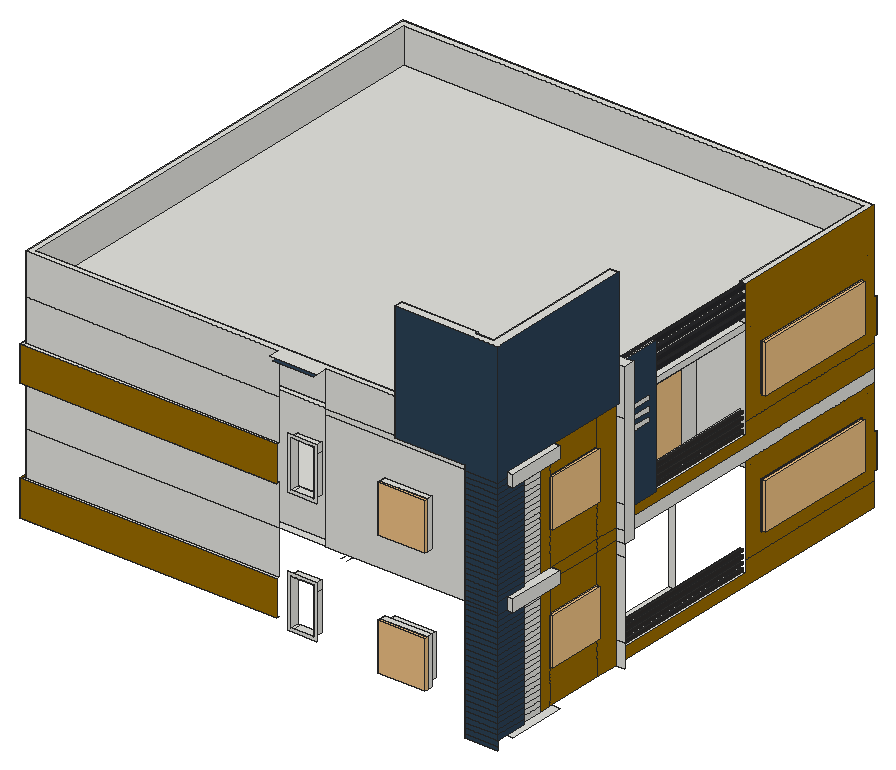
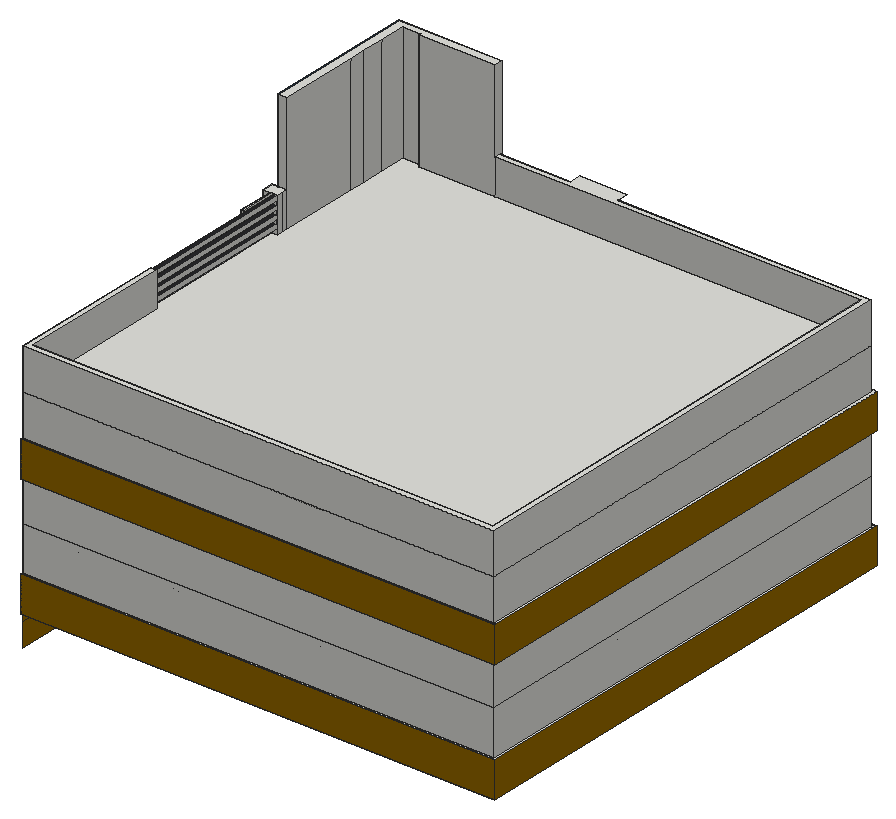
# SketchUp Ruby script. Lengths in inches.
U = 1.inch
M = Sketchup.active_model
def pt(a) = Geom::Point3d.new(a.map { |v| v * U })
def face(e, loops, mat)
  f = e.add_face(loops[0].map { |a| pt(a) })
  loops[1..].each { |l| e.add_face(l.map { |a| pt(a) }).erase! }
  f.material = f.back_material = mat if mat
  f
end
# faces: each face lists its corners as indices into pts; further lists are holes
def faces(e, pts, list, mat = nil) = list.each { |f| face(e, (f[0].is_a?(Array) ? f : [f]).map { |l| l.map { |i| pts[i] } }, mat) }
# xy, xz, yz: faces in a plane at the given z, y or x. An outline is a flat list of corners, or four numbers for a rectangle; further outlines are holes
def ring(l) = l.size == 4 ? [[l[0], l[1]], [l[2], l[1]], [l[2], l[3]], [l[0], l[3]]] : l.each_slice(2).to_a
def flat(e, list, mat, &to3) = list.each { |f| face(e, (f[0].is_a?(Array) ? f : [f]).map { |l| ring(l).map { |u, v| to3.(u, v) } }, mat) }
def xy(e, z, list, mat = nil) = flat(e, list, mat) { |x, y| [x, y, z] }
def xz(e, y, list, mat = nil) = flat(e, list, mat) { |x, z| [x, y, z] }
def yz(e, x, list, mat = nil) = flat(e, list, mat) { |y, z| [x, y, z] }
def lines(e, pts, list) = list.each { |a, b| e.add_line(pt(pts[a]), pt(pts[b])) }
# prism: a flat outline (further loops are holes) pulled along v
def prism(e, loops, v, mat = nil)
  f = face(e, loops, mat); d = Geom::Vector3d.new(v.map { |x| x * U })
  f.pushpull(f.normal.samedirection?(d) ? d.length : -d.length)
end
def box(e, o, s, mat = nil) = prism(e, [[o, [o[0] + s[0], o[1], o[2]], [o[0] + s[0], o[1] + s[1], o[2]], [o[0], o[1] + s[1], o[2]]]], [0, 0, s[2]], mat)
def at(x, y, z, deg = 0) = Geom::Transformation.translation(pt([x, y, z])) * Geom::Transformation.rotation(ORIGIN, Z_AXIS, deg.degrees)
def axes(o, x, y, z) = Geom::Transformation.new([*x, 0, *y, 0, *z, 0, *pt(o).to_a, 1])
def part(name) = M.definitions.add(name)
# library, detail: a bought-in or finely detailed component or shape, given as its bounding box
def library(name, o, s) = part(name).tap { |d| box(d.entities, o, s) }
def detail(e, o, s) = box(e.add_group.entities, o, s)
def put(e, d, t, mat = nil) = e.add_instance(d, t).tap { |i| i.material = mat if mat }
def group(e, t, mat = nil) = e.add_group.tap { |g| g.transformation = t; g.material = mat if mat }.entities
root = M.entities
M.materials.add("Carpet_04_1K").color = [43, 65, 85]
M.materials.add("D07_Ochre_Flame").color = [153, 107, 0]
M.materials.add("ThomThom - Buttons2").color = [40, 40, 43]
M.materials.add("ThomThom - Hat1").color = [48, 46, 44]
c1 = library("mesh-163",[-551.08,-704.17,-20.03],[1929.24,1401.85,86.96])
c2 = part("Group11")
put(c2.entities,c1,at(0,0,0))
xy(root,387,[[426,202,432,302]])
xy(root,396,[[486,21.29,492,21.29,492,81.29,483,81.29,483,42,486,42]])
xy(root,408,[[474,175,477,329],[480,175,483,329]])
xy(root,411,[[477,175,480,329]],"ThomThom - Hat1")
xy(root,414,[[477,175,480,329]])
xy(root,417,[[477,175,480,329]],"ThomThom - Hat1")
xy(root,420,[[369,6,417,12],[477,175,480,329]])
xy(root,423,[[372,6,414,21],[273,12,276,21],[276,12,297,21]])
xy(root,423,[[477,175,480,329]],"ThomThom - Hat1")
xy(root,426,[[477,175,480,329]])
xy(root,429,[[0,9,261,12],[0,12,3,495],[3,492,483,495]])
xy(root,429,[[477,175,480,329]],"ThomThom - Hat1")
xy(root,435,[[474,82,483,136]])
xy(root,438,[[483,347,485,474]])
xy(root,441,[[474,350,485,471]])
xy(root,465,[[372,6,414,21],[0,9,261,12],[0,12,3,495],[3,492,483,495]])
xy(root,468,[[369,6,417,12]])
xy(root,471,[[273,12,297,21]])
xy(root,477,[[474,82,483,136],[426,202,432,302]])
xy(root,483,[[474,350,485,471]])
xy(root,486,[[483,347,485,474]])
xy(root,504,[[12,21,171,169],[180,21,324,169],[330,21,474,169],[171,169,180,175],[180,169,324,175],
  [324,169,330,175],[12,175,171,329],[171,175,180,329],[180,175,324,329],[324,175,330,329],
  [330,175,426,329],[171,329,180,335],[180,329,324,335],[324,329,330,335],[330,329,426,335],
  [12,335,171,483],[171,335,180,483],[180,335,324,483],[324,335,330,483],[330,335,426,483],
  [426,335,474,483]])
xy(root,510,[[180,21,324,169],[330,21,474,169],[486,21.29,486,42,483,42,483,81.29,492,81.29,492,21.29],[12,175,426,329],[432,175,474,329],
  [12,335,474,483]])
xy(root,510,[[12,21,171,169]],"D07_Ochre_Flame")
xy(root,513,[[426,202,432,302]])
xy(root,522,[[486,21.29,492,21.29,492,81.29,483,81.29,483,42,486,42]])
xy(root,534,[[474,175,477,329],[480,175,483,329],[483,175,485.29,211]])
xy(root,537,[[477,175,480,329]],"ThomThom - Hat1")
xy(root,540,[[477,175,480,329]])
xy(root,543,[[477,175,480,329]],"ThomThom - Hat1")
xy(root,546,[[369,6,417,12],[477,175,480,329]])
xy(root,549,[[372,6,414,21],[273,12,276,21],[276,12,297,21]])
xy(root,549,[[477,175,480,329]],"ThomThom - Hat1")
xy(root,552,[[0,9,3,492],[3,9,261,12],[477,175,480,329],[0,492,483,495]])
xy(root,555,[[477,175,480,329]],"ThomThom - Hat1")
xy(root,561,[[474,82,483,136]])
xy(root,564,[[483,347,485,474]])
xy(root,567,[[474,350,485,471]])
xy(root,588,[[0,9,3,492],[3,9,261,12],[0,492,483,495]])
xy(root,591,[[372,6,414,21]])
xy(root,594,[[369,6,417,12]])
xy(root,597,[[273,12,297,21]])
xy(root,603,[[474,82,483,136],[426,202,432,302]])
xy(root,609,[[474,350,485,471]])
xy(root,612,[[483,347,485,474]])
xy(root,624,[[486,21.29,486,42,483,42,483,81.29,492,81.29,492,21.29]])
xy(root,624,[[483,21.29,486,42]],"Carpet_04_1K")
xy(root,630,[[12,21,171,169],[180,21,324,169],[330,21,474,169],[171,169,180,175],[180,169,324,175],
  [324,169,330,175],[12,175,171,329],[171,175,180,329],[180,175,324,329],[324,175,330,329],
  [330,175,426,329],[432,175,483,329],[171,329,180,335],[180,329,324,335],[324,329,330,335],
  [330,329,426,335],[12,335,171,483],[171,335,180,483],[180,335,324,483],[324,335,330,483],
  [330,335,426,483],[426,335,474,483],[171,483,180,492],[180,483,324,492],[324,483,330,492],
  [330,483,426,492]])
xy(root,636,[[459,15,477,15,477,175,483,175,483,329,477,329,477,486,9,486,9,18,459,18],[486,21.29,492,81.29]])
xy(root,636,[[381,9,453,12]],"Carpet_04_1K")
xy(root,636,[[483,21.29,486,81.29],[483,81.29,486,163]],"D07_Ochre_Flame")
xy(root,641.25,[[478,175,482,329]])
xy(root,645.5,[[478,175,482,329]],"ThomThom - Buttons2")
xy(root,649.75,[[478,175,482,329]])
xy(root,654,[[478,175,482,329]],"ThomThom - Buttons2")
xy(root,658.25,[[478,175,482,329]])
xy(root,662.5,[[478,175,482,329]],"ThomThom - Buttons2")
xy(root,666.75,[[478,175,482,329]])
xy(root,669,[[264,0,306,12]],"Carpet_04_1K")
xy(root,671,[[478,175,482,329]],"ThomThom - Buttons2")
xy(root,672,[[261,0,309,0,309,12,381,12,381,18,9,18,9,486,477,486,477,329,483,329,483,492,3,492,3,12,261,12],[477,163,492,163,492,175,485.29,175,485.29,211,483,211,483,175,477,175]])
xy(root,756,[[381,9,486,9,486,163,477,163,477,15,459,15,459,18,381,18]])
xz(root,6,[[[369,420,417,468],[372,423,414,465]],[[369,546,417,594],[372,549,414,591]]])
xz(root,9,[[453,387.3125,486,390.625],[453,390.625,486,396],[453,396,486,401.18],[453,401.18,486,406.36],[453,406.36,486,411.55],
  [453,411.55,486,416.73],[453,416.73,486,421.91],[453,421.91,486,427.09],[453,427.09,486,432.27],[453,432.27,486,437.45],
  [453,437.45,486,442.64],[453,442.64,486,447.82],[453,447.82,486,453],[453,453,486,458.18],[453,458.18,486,463.36],
  [453,463.36,486,468.55],[453,468.55,486,473.73],[453,473.73,486,478.91],[453,478.91,486,484.09],[453,484.09,486,489.27],
  [453,489.27,486,494.45],[453,494.45,486,499.64],[453,499.64,486,504.82],[453,504.82,486,510],[453,510,486,513.3125],
  [453,513.3125,486,516.625],[453,516.625,486,522],[453,522,486,527.18],[453,527.18,486,532.36],[453,532.36,486,537.55],
  [453,537.55,486,542.73],[453,542.73,486,547.91],[453,547.91,486,553.09],[453,553.09,486,558.27],[453,558.27,486,563.45],
  [453,563.45,486,568.64],[453,568.64,486,573.82],[453,573.82,486,579],[453,579,486,584.18],[453,584.18,486,589.36],
  [453,589.36,486,594.55],[453,594.55,486,599.73],[453,599.73,486,604.91],[453,604.91,486,610.09],[453,610.09,486,615.27],
  [453,615.27,486,620.45],[453,620.45,486,625.64],[453,625.64,486,630.82],[453,630.82,486,630.82,486,756,381,756,381,636,453,636]],"Carpet_04_1K")
xz(root,9,[[0,429,261,465],[0,552,261,588]],"D07_Ochre_Flame")
xz(root,12,[[[270,420,300,474],[273,423,297,471]],[3,465,261,510],[3,510,261,552],[[309,510,453,630],[369,546,417,594]],[[270,546,300,600],[273,549,297,597]],
  [3,588,261,630],[3,630,261,672],[309,630,453,636],[309,636,381,672]])
xz(root,15,[[459,636,477,756]])
xz(root,18,[[9,636,381,672],[381,636,459,756]])
xz(root,21,[[12,510,171,630],[[180,510,324,630],[273,549,297,597]],[[330,510,474,630],[372,549,414,591]]])
xz(root,21.29,[[486,510,492,522],[486,624,492,636]])
xz(root,21.29,[[483,624,486,625.64],[483,625.64,486,630.82],[483,630.82,486,636]],"Carpet_04_1K")
xz(root,42,[[483,396,486,401.18],[483,401.18,486,406.36],[483,406.36,486,411.55],[483,411.55,486,416.73],[483,416.73,486,421.91],
  [483,421.91,486,427.09],[483,427.09,486,432.27],[483,432.27,486,437.45],[483,437.45,486,442.64],[483,442.64,486,447.82],
  [483,447.82,486,453],[483,453,486,458.18],[483,458.18,486,463.36],[483,463.36,486,468.55],[483,468.55,486,473.73],
  [483,473.73,486,478.91],[483,478.91,486,484.09],[483,484.09,486,489.27],[483,489.27,486,494.45],[483,494.45,486,498],
  [483,522,486,527.18],[483,527.18,486,532.36],[483,532.36,486,537.55],[483,537.55,486,542.73],[483,542.73,486,547.91],
  [483,547.91,486,553.09],[483,553.09,486,558.27],[483,558.27,486,563.45],[483,563.45,486,568.64],[483,568.64,486,573.82],
  [483,573.82,486,579],[483,579,486,584.18],[483,584.18,486,589.36],[483,589.36,486,594.55],[483,594.55,486,599.73],
  [483,599.73,486,604.91],[483,604.91,486,610.09],[483,610.09,486,615.27],[483,615.27,486,620.45],[483,620.45,486,624]])
xz(root,42,[[483,498,486,499.64],[483,499.64,486,504.82],[483,504.82,486,510]],"Carpet_04_1K")
xz(root,81.29,[[483,510,492,522],[483,624,492,636]])
xz(root,82,[[474,435,483,477],[474,561,483,603]])
xz(root,136,[[474,435,483,477],[474,561,483,603]])
xz(root,163,[[483,396,492,420],[483,420,492,498],[483,498,492,510],[483,510,492,522],[483,522,492,546],
  [483,546,492,624],[483,624,492,624,492,672,486,672,486,636,483,636],[483,636,486,672],[477,672,486,756]])
xz(root,169,[[12,510,171,630],[171,510,180,630],[180,510,324,630],[324,510,330,630],[330,510,474,630]])
xz(root,175,[[12,510,426,630],[[432,510,432,630,483,630,483,534,480,534,480,537,477,537,477,534,474,534,474,510],[477,552,480,555],[477,540,480,543],[477,546,480,549]],[483,510,492,522],[483,522,492,534],[485.29,534,492,672],
  [[477,636,483,672],[478,666.75,482,671],[478,658.25,482,662.5],[478,649.75,482,654],[478,641.25,482,645.5]]])
xz(root,202,[[426,387,432,477],[426,513,432,603]])
xz(root,211,[[483,534,485.29,672]])
xz(root,302,[[426,387,432,477],[426,513,432,603]])
xz(root,329,[[432,504,483,510],[12,510,426,630],[[432,510,474,510,474,534,477,534,477,537,480,537,480,534,483,534,483,630,432,630],[477,540,480,543],[477,546,480,549],[477,552,480,555]],[[477,636,483,672],[478,666.75,482,671],[478,641.25,482,645.5],[478,658.25,482,662.5],[478,649.75,482,654]]])
xz(root,335,[[12,510,474,630]])
xz(root,347,[[483,438,485,486],[483,564,485,612]])
xz(root,350,[[474,441,485,483],[474,567,485,609]])
xz(root,471,[[474,441,485,483],[474,567,485,609]])
xz(root,474,[[483,438,485,486],[483,564,485,612]])
xz(root,483,[[12,510,474,630]])
xz(root,486,[[9,636,477,672]])
xz(root,492,[[3,465,483,510],[3,510,483,552],[3,588,483,630],[3,630,483,672]])
xz(root,495,[[0,429,483,465],[0,552,483,588]],"D07_Ochre_Flame")
yz(root,0,[[9,429,495,465],[9,552,495,588]],"D07_Ochre_Flame")
yz(root,3,[[12,465,492,510],[12,510,492,552],[12,588,492,630],[12,630,492,672]])
yz(root,9,[[18,636,486,672]])
yz(root,12,[[21,510,169,630],[175,510,329,630],[335,510,483,630]])
yz(root,171,[[21,510,169,630]])
yz(root,180,[[21,510,169,630]])
yz(root,273,[[12,423,21,471],[12,549,21,597]])
yz(root,297,[[12,423,21,462],[12,462,21,471],[12,549,21,588],[12,588,21,597]])
yz(root,324,[[21,510,169,630]])
yz(root,330,[[21,510,169,630]])
yz(root,369,[[6,420,12,468],[6,546,12,594]])
yz(root,372,[[6,423,21,465],[6,549,21,591]])
yz(root,381,[[9,672,18,756]])
yz(root,381,[[9,636,12,672]],"Carpet_04_1K")
yz(root,414,[[6,423,21,465],[6,549,21,591]])
yz(root,417,[[6,420,12,468],[6,546,12,594]])
yz(root,426,[[[175,510,329,630],[202,513,302,603]]])
yz(root,432,[[175,504,329,510],[175,510,199,510,199,606,305,606,305,510,329,510,329,630,175,630],[[199,510,305,606],[202,513,302,603]]])
yz(root,453,[[9,387.3125,12,390.625],[9,390.625,12,396],[9,396,12,401.18],[9,401.18,12,406.36],[9,406.36,12,411.55],
  [9,411.55,12,416.73],[9,416.73,12,421.91],[9,421.91,12,427.09],[9,427.09,12,432.27],[9,432.27,12,437.45],
  [9,437.45,12,442.64],[9,442.64,12,447.82],[9,447.82,12,453],[9,453,12,458.18],[9,458.18,12,463.36],
  [9,463.36,12,468.55],[9,468.55,12,473.73],[9,473.73,12,478.91],[9,478.91,12,484.09],[9,484.09,12,489.27],
  [9,489.27,12,494.45],[9,494.45,12,499.64],[9,499.64,12,504.82],[9,504.82,12,510],[9,510,12,513.3125],
  [9,513.3125,12,516.625],[9,516.625,12,522],[9,522,12,527.18],[9,527.18,12,532.36],[9,532.36,12,537.55],
  [9,537.55,12,542.73],[9,542.73,12,547.91],[9,547.91,12,553.09],[9,553.09,12,558.27],[9,558.27,12,563.45],
  [9,563.45,12,568.64],[9,568.64,12,573.82],[9,573.82,12,579],[9,579,12,584.18],[9,584.18,12,589.36],
  [9,589.36,12,594.55],[9,594.55,12,599.73],[9,599.73,12,604.91],[9,604.91,12,610.09],[9,610.09,12,615.27],
  [9,615.27,12,620.45],[9,620.45,12,625.64],[9,625.64,12,630.82],[9,630.82,12,636]])
yz(root,459,[[15,636,18,756]])
yz(root,474,[[[21,510,169,630],[82,561,136,603]],[175,510,329,534],[[335,510,483,630],[350,567,471,609]]])
yz(root,477,[[175,408,329,411],[175,414,329,417],[175,420,329,423],[175,426,329,429],[175,534,329,537],
  [175,540,329,543],[175,546,329,549],[175,552,329,555],[15,636,42,756],[42,636,66,756],
  [66,636,81.29,756],[81.29,636,163,756],[163,636,169,672],[169,636,175,672],[329,636,486,672]])
yz(root,478,[[175,641.25,329,645.5],[175,649.75,329,654],[175,658.25,329,662.5],[175,666.75,329,671]])
yz(root,480,[[175,408,329,411],[175,414,329,417],[175,420,329,423],[175,426,329,429],[175,534,329,537],
  [175,540,329,543],[175,546,329,549],[175,552,329,555]],"ThomThom - Hat1")
yz(root,482,[[175,641.25,329,645.5],[175,649.75,329,654],[175,658.25,329,662.5],[175,666.75,329,671]],"ThomThom - Buttons2")
yz(root,483,[[42,396,66,401.18],[42,401.18,66,406.36],[42,406.36,66,411.55],[42,411.55,66,416.73],[42,416.73,66,421.91],
  [42,421.91,66,427.09],[42,427.09,66,432.27],[[79,432,139,480],[82,435,136,477]],[42,432.27,66,437.45],[42,437.45,66,442.64],
  [42,442.64,66,447.82],[42,447.82,66,453],[42,453,66,458.18],[42,458.18,66,463.36],[42,463.36,66,468.55],
  [42,468.55,66,473.73],[42,473.73,66,478.91],[42,478.91,66,484.09],[42,484.09,66,489.27],[42,489.27,66,494.45],
  [42,494.45,66,499.64],[42,499.64,66,504.82],[42,504.82,66,510],[79,510,81.29,522],[175,510,492,522],
  [42,522,66,527.18],[42,527.18,66,532.36],[42,532.36,66,537.55],[175,534,211,630],[42,537.55,66,542.73],
  [42,542.73,66,547.91],[42,547.91,66,553.09],[42,553.09,66,558.27],[[79,558,139,606],[82,561,136,603]],[42,558.27,66,563.45],
  [42,563.45,66,568.64],[42,568.64,66,573.82],[42,573.82,66,579],[42,579,66,584.18],[42,584.18,66,589.36],
  [42,589.36,66,594.55],[42,594.55,66,599.73],[42,599.73,66,604.91],[42,604.91,66,610.09],[42,610.09,66,615.27],
  [42,615.27,66,620.45],[42,620.45,66,624],[211,630,329,636],[175,636,211,672]])
yz(root,483,[[21.29,624,81.29,625.64],[21.29,625.64,81.29,630.82],[21.29,630.82,81.29,636]],"Carpet_04_1K")
yz(root,483,[[66,396,79,510],[79,396,139,432],[139,396,163,510],[175,396,492,396,492,420,329,420,329,408,175,408],[[329,420,492,420,492,429,495,429,495,465,492,465,492,510,329,510],[347,438,474,486]],
  [79,480,139,510],[81.29,510,139,522],[139,510,163,522],[66,522,79,624],[79,522,139,558],
  [139,522,163,636],[175,522,492,522,492,546,329,546,329,534,175,534],[[329,546,492,546,492,552,495,552,495,588,492,588,492,672,329,672],[347,564,474,612]],[79,606,139,606,139,636,81.29,636,81.29,624,79,624]],"D07_Ochre_Flame")
yz(root,485,[[[347,438,474,486],[350,441,471,483]],[[347,564,474,612],[350,567,471,609]]])
yz(root,485.29,[[183.67,601.29,203.72,607.21],[183.67,610.93,203.72,616.85],[183.67,621.19,203.72,627.11]])
yz(root,485.29,[[[175,534,211,672],[183.67,621.19,203.72,627.11],[183.67,610.93,203.72,616.85],[183.67,601.29,203.72,607.21]]],"Carpet_04_1K")
yz(root,486,[[9,396,42,401.18],[9,401.18,42,406.36],[9,406.36,42,411.55],[9,411.55,42,416.73],[9,416.73,42,421.91],
  [9,421.91,42,427.09],[9,427.09,42,432.27],[9,432.27,42,437.45],[9,437.45,42,442.64],[9,442.64,42,447.82],
  [9,447.82,42,453],[9,453,42,458.18],[9,458.18,42,463.36],[9,463.36,42,468.55],[9,468.55,42,473.73],
  [9,473.73,42,478.91],[9,478.91,42,484.09],[9,484.09,42,489.27],[9,489.27,42,494.45],[9,494.45,42,499.64],
  [9,499.64,42,504.82],[9,504.82,42,510],[9,510,21.29,522],[9,522,42,527.18],[9,527.18,42,532.36],
  [9,532.36,42,537.55],[9,537.55,42,542.73],[9,542.73,42,547.91],[9,547.91,42,553.09],[9,553.09,42,558.27],
  [9,558.27,42,563.45],[9,563.45,42,568.64],[9,568.64,42,573.82],[9,573.82,42,579],[9,579,42,584.18],
  [9,584.18,42,589.36],[9,589.36,42,594.55],[9,594.55,42,599.73],[9,599.73,42,604.91],[9,604.91,42,610.09],
  [9,610.09,42,615.27],[9,615.27,42,620.45],[9,620.45,42,620.45,42,624,21.29,624,21.29,625.64,9,625.64],[9,625.64,21.29,630.82],[9,630.82,21.29,630.82,21.29,636,163,636,163,756,9,756]],"Carpet_04_1K")
yz(root,492,[[21.29,510,81.29,522],[163,510,175,672],[21.29,624,81.29,636]])
p = [[324,21,504],[324,12,504],[330,21,504],[330,12,504],[474,21,504],[474,12,504],
  [474,169,504],[474,175,504],[426,483,504],[426,492,504],[330,483,504],[330,492,504],
  [324,483,504],[324,492,504],[180,483,504],[180,492,504],[474,483,504],[483,483,504],
  [474,335,504],[483,335,504],[12,335,504],[3,335,504],[477,329,411],[477,329,414],
  [477,175,411],[477,175,414],[477,329,417],[477,329,420],[477,175,417],[477,175,420],
  [477,329,423],[477,329,426],[477,175,423],[477,175,426],[324,21,630],[324,12,630],
  [330,21,630],[330,12,630],[474,21,630],[474,12,630],[474,169,630],[474,175,630],
  [474,483,630],[483,483,630],[474,335,630],[483,335,630],[12,335,630],[3,335,630],
  [12,175,630],[3,175,630],[12,169,630],[3,169,630],[12,21,630],[3,21,630],
  [477,329,537],[477,329,540],[477,175,537],[477,175,540],[477,329,543],[477,329,546],
  [477,175,543],[477,175,546],[477,329,549],[477,329,552],[477,175,549],[477,175,552],
  [3,492,570],[485,474,564],[478,175,662.5],[478,175,666.75],[478,329,662.5],[478,329,666.75],
  [478,175,654],[478,175,658.25],[478,329,654],[478,329,658.25],[478,175,645.5],[478,175,649.75],
  [478,329,645.5],[478,329,649.75]]
lines(root,p,[[0,1],[2,3],[4,5],[6,7],[8,9],[10,11],[12,13],[14,15],[16,17],[18,19],[20,21],[22,23],
  [24,25],[26,27],[28,29],[30,31],[32,33],[34,35],[36,37],[38,39],[40,41],[42,43],[44,45],[46,47],
  [48,49],[50,51],[52,53],[54,55],[56,57],[58,59],[60,61],[62,63],[64,65],[66,67],[68,69],[70,71],
  [72,73],[74,75],[76,77],[78,79]])
put(root,c2,axes([382.72,5.21,444.14],[0.0249,0,0],[0,0,0.0342],[0,-0.03937,0]))
put(root,c2,axes([483.79,96.09,456.1],[0,0.03102,0],[0,0,0.03425],[0.03937,0,0]))
put(root,c2,axes([485.79,383.02,462.65],[0,0.06535,0],[0,0,0.03346],[0.03937,0,0]))
put(root,c2,axes([432.79,229.375,558.22],[0,0.05512,0],[0,0,0.06848],[0.03937,0,0]))
put(root,c2,axes([382.71,5.21,570.11],[0.02488,0,0],[0,0,0.03424],[0,-0.03937,0]))
put(root,c2,axes([483.79,95.92,582.1],[0,0.03071,0],[0,0,0.03425],[0.03937,0,0]))
put(root,c2,axes([485.79,383.28,587.83],[0,0.06583,0],[0,0,0.03465],[0.03937,0,0]))
